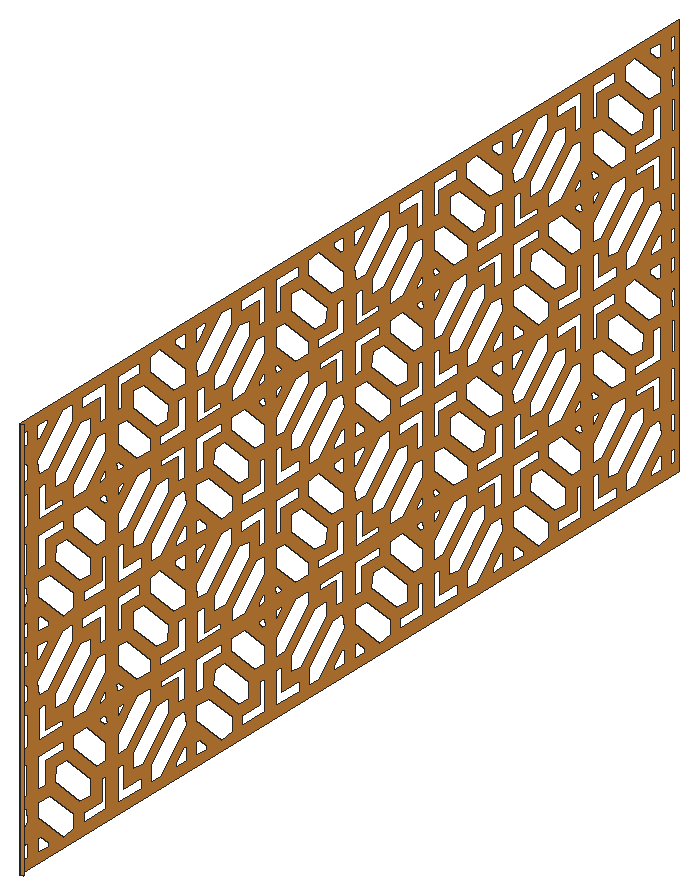
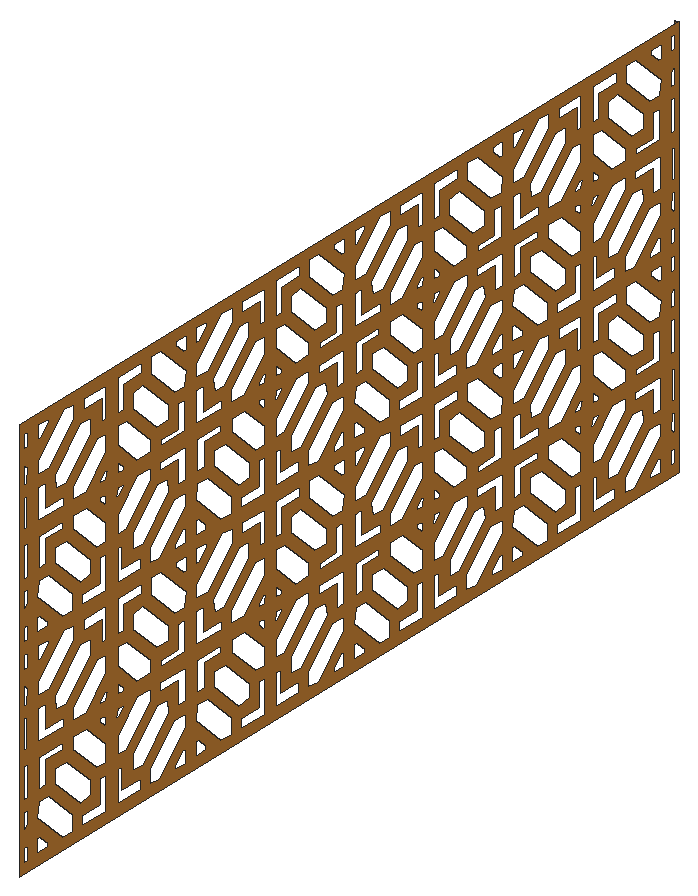
# SketchUp Ruby script. Lengths in inches.
U = 1.inch
M = Sketchup.active_model
def pt(a) = Geom::Point3d.new(a.map { |v| v * U })
def face(e, loops, mat)
  f = e.add_face(loops[0].map { |a| pt(a) })
  loops[1..].each { |l| e.add_face(l.map { |a| pt(a) }).erase! }
  f.material = f.back_material = mat if mat
  f
end
# faces: each face lists its corners as indices into pts; further lists are holes
def faces(e, pts, list, mat = nil) = list.each { |f| face(e, (f[0].is_a?(Array) ? f : [f]).map { |l| l.map { |i| pts[i] } }, mat) }
# xy, xz, yz: faces in a plane at the given z, y or x. An outline is a flat list of corners, or four numbers for a rectangle; further outlines are holes
def ring(l) = l.size == 4 ? [[l[0], l[1]], [l[2], l[1]], [l[2], l[3]], [l[0], l[3]]] : l.each_slice(2).to_a
def flat(e, list, mat, &to3) = list.each { |f| face(e, (f[0].is_a?(Array) ? f : [f]).map { |l| ring(l).map { |u, v| to3.(u, v) } }, mat) }
def xy(e, z, list, mat = nil) = flat(e, list, mat) { |x, y| [x, y, z] }
def xz(e, y, list, mat = nil) = flat(e, list, mat) { |x, z| [x, y, z] }
def yz(e, x, list, mat = nil) = flat(e, list, mat) { |y, z| [x, y, z] }
def lines(e, pts, list) = list.each { |a, b| e.add_line(pt(pts[a]), pt(pts[b])) }
# prism: a flat outline (further loops are holes) pulled along v
def prism(e, loops, v, mat = nil)
  f = face(e, loops, mat); d = Geom::Vector3d.new(v.map { |x| x * U })
  f.pushpull(f.normal.samedirection?(d) ? d.length : -d.length)
end
def box(e, o, s, mat = nil) = prism(e, [[o, [o[0] + s[0], o[1], o[2]], [o[0] + s[0], o[1] + s[1], o[2]], [o[0], o[1] + s[1], o[2]]]], [0, 0, s[2]], mat)
def at(x, y, z, deg = 0) = Geom::Transformation.translation(pt([x, y, z])) * Geom::Transformation.rotation(ORIGIN, Z_AXIS, deg.degrees)
def axes(o, x, y, z) = Geom::Transformation.new([*x, 0, *y, 0, *z, 0, *pt(o).to_a, 1])
def part(name) = M.definitions.add(name)
# library, detail: a bought-in or finely detailed component or shape, given as its bounding box
def library(name, o, s) = part(name).tap { |d| box(d.entities, o, s) }
def detail(e, o, s) = box(e.add_group.entities, o, s)
def put(e, d, t, mat = nil) = e.add_instance(d, t).tap { |i| i.material = mat if mat }
def group(e, t, mat = nil) = e.add_group.tap { |g| g.transformation = t; g.material = mat if mat }.entities
root = M.entities
M.materials.add("1056 AP 9903 Mellow Melon-N").color = [219, 142, 59]
xz(root,13.79,[[14.35,145.75,15.0625,238.4375]],"1056 AP 9903 Mellow Melon-N")
yz(root,14.35,[[[13.79,145.75,202.3125,238.4375],[94.27,153.04,101.6,160.37,101.6,163.43,98.2,163.43,91.29,156.53,91.29,153.47],[94.27,198.38,101.6,205.71,101.6,208.78,98.2,208.78,91.29,201.875,91.29,198.8125],[23.81,175.41,27.21,175.41,34.12,182.3125,34.12,185.375,31.14,185.81,23.81,178.47],[69.15,175.41,72.56,175.41,79.46,182.3125,79.46,185.375,76.48,185.81,69.15,178.47],[69.15,220.75,72.56,220.75,79.46,227.66,79.46,230.72,76.48,231.15,69.15,223.82],[23.81,220.75,27.21,220.75,34.12,227.66,34.12,230.72,31.14,231.15,23.81,223.82],[159.84,220.75,163.24,220.75,170.15,227.66,170.15,230.72,167.17,231.15,159.84,223.82],[159.84,175.41,163.24,175.41,170.15,182.3125,170.15,185.375,167.17,185.81,159.84,178.47],[48.93,153.04,56.26,160.37,56.26,163.43,52.85,163.43,45.95,156.53,45.95,153.47],[48.93,198.38,56.26,205.71,56.26,208.78,52.85,208.78,45.95,201.875,45.95,198.8125],[184.96,153.04,192.29,160.37,192.29,163.43,188.88,163.43,181.98,156.53,181.98,153.47],[139.62,153.04,146.95,160.37,146.95,163.43,143.54,163.43,136.64,156.53,136.64,153.47],[114.49,220.75,117.9,220.75,124.81,227.66,124.81,230.72,121.83,231.15,114.49,223.82],[114.49,175.41,117.9,175.41,124.81,182.3125,124.81,185.375,121.83,185.81,114.49,178.47],[139.62,198.38,146.95,205.71,146.95,208.78,143.54,208.78,136.64,201.875,136.64,198.8125],[184.96,198.38,192.29,205.71,192.29,208.78,188.88,208.78,181.98,201.875,181.98,198.8125],[98.27,175.34,101.33,175.34,101.76,178.32,94.43,185.65,91.36,185.65,91.36,182.24],[98.27,220.68,101.33,220.68,101.76,223.66,94.43,230.99,91.36,230.99,91.36,227.59],[52.92,175.34,55.99,175.34,56.42,178.32,49.09,185.65,46.02,185.65,46.02,182.24],[143.61,175.34,146.68,175.34,147.1,178.32,139.77,185.65,136.71,185.65,136.71,182.24],[30.98,198.54,34.05,198.54,34.05,201.95,27.14,208.85,24.08,208.85,23.65,205.87],[76.32,198.54,79.39,198.54,79.39,201.95,72.49,208.85,69.42,208.85,68.99,205.87],[52.92,220.68,55.99,220.68,56.42,223.66,49.09,230.99,46.02,230.99,46.02,227.59],[30.98,153.19,34.05,153.19,34.05,156.6,27.14,163.51,24.08,163.51,23.65,160.53],[76.32,153.19,79.39,153.19,79.39,156.6,72.49,163.51,69.42,163.51,68.99,160.53],[143.61,220.68,146.68,220.68,147.1,223.66,139.77,230.99,136.71,230.99,136.71,227.59],[188.96,175.34,192.02,175.34,192.45,178.32,185.12,185.65,182.05,185.65,182.05,182.24],[121.67,198.54,124.73,198.54,124.73,201.95,117.83,208.85,114.77,208.85,114.34,205.87],[167.01,198.54,170.08,198.54,170.08,201.95,163.17,208.85,160.11,208.85,159.68,205.87],[188.96,220.68,192.02,220.68,192.45,223.66,185.12,230.99,182.05,230.99,182.05,227.59],[121.67,153.19,124.73,153.19,124.73,156.6,117.83,163.51,114.77,163.51,114.34,160.53],[167.01,153.19,170.08,153.19,170.08,156.6,163.17,163.51,160.11,163.51,159.68,160.53],[96.45,148.27,99.42,148.27,106.76,155.61,106.33,158.67,103.35,158.67,96.45,151.76],[141.79,148.27,144.77,148.27,152.11,155.61,151.67,158.67,148.7,158.67,141.79,151.76],[96.45,193.61,99.42,193.61,106.76,200.95,106.33,204.01,103.35,204.01,96.45,197.11],[141.79,193.61,144.77,193.61,152.11,200.95,151.67,204.01,148.7,204.01,141.79,197.11],[187.14,148.27,190.11,148.27,197.45,155.61,197.02,158.67,194.04,158.67,187.14,151.76],[51.11,148.27,54.08,148.27,61.42,155.61,60.99,158.67,58.01,158.67,51.11,151.76],[187.14,193.61,190.11,193.61,197.45,200.95,197.02,204.01,194.04,204.01,187.14,197.11],[51.11,193.61,54.08,193.61,61.42,200.95,60.99,204.01,58.01,204.01,51.11,197.11],[193.72,180.49,197.22,180.49,197.22,183.47,189.88,190.81,186.82,190.375,186.82,187.4],[193.72,225.84,197.22,225.84,197.22,228.8125,189.88,236.15,186.82,235.72,186.82,232.74],[26.22,193.38,29.28,193.8125,29.28,196.79,22.375,203.69,18.88,203.69,18.88,200.72],[116.91,193.38,119.97,193.8125,119.97,196.79,113.0625,203.69,109.57,203.69,109.57,200.72],[162.25,193.38,165.3125,193.8125,165.3125,196.79,158.41,203.69,154.91,203.69,154.91,200.72],[71.5625,193.38,74.625,193.8125,74.625,196.79,67.72,203.69,64.22,203.69,64.22,200.72],[71.5625,148.03,74.625,148.47,74.625,151.45,67.72,158.35,64.22,158.35,64.22,155.375],[26.22,148.03,29.28,148.47,29.28,151.45,22.375,158.35,18.88,158.35,18.88,155.375],[116.91,148.03,119.97,148.47,119.97,151.45,113.0625,158.35,109.57,158.35,109.57,155.375],[162.25,148.03,165.3125,148.47,165.3125,151.45,158.41,158.35,154.91,158.35,154.91,155.375],[103.04,225.84,106.53,225.84,106.53,228.8125,99.19,236.15,96.13,235.72,96.13,232.74],[103.04,180.49,106.53,180.49,106.53,183.47,99.19,190.81,96.13,190.375,96.13,187.4],[148.38,225.84,151.875,225.84,151.875,228.8125,144.54,236.15,141.48,235.72,141.48,232.74],[148.38,180.49,151.875,180.49,151.875,183.47,144.54,190.81,141.48,190.375,141.48,187.4],[57.69,225.84,61.1875,225.84,61.1875,228.8125,53.85,236.15,50.79,235.72,50.79,232.74],[57.69,180.49,61.1875,180.49,61.1875,183.47,53.85,190.81,50.79,190.375,50.79,187.4],[109.77,180.18,112.75,180.18,119.65,187.08,119.65,190.58,116.67,190.58,109.33,183.24],[109.77,225.52,112.75,225.52,119.65,232.42,119.65,235.92,116.67,235.92,109.33,228.58],[155.11,225.52,158.09,225.52,164.99,232.42,164.99,235.92,162.02,235.92,154.68,228.58],[155.11,180.18,158.09,180.18,164.99,187.08,164.99,190.58,162.02,190.58,154.68,183.24],[64.42,225.52,67.4,225.52,74.31,232.42,74.31,235.92,71.33,235.92,63.99,228.58],[64.42,180.18,67.4,180.18,74.31,187.08,74.31,190.58,71.33,190.58,63.99,183.24],[19.08,180.18,22.06,180.18,28.96,187.08,28.96,190.58,25.99,190.58,18.65,183.24],[19.08,225.52,22.06,225.52,28.96,232.42,28.96,235.92,25.99,235.92,18.65,228.58],[28.96,216.42,32.8,216.42,38.41,222.03,38.41,225.95,35.87,225.95,28.96,219.05],[74.31,216.42,78.15,216.42,83.76,222.03,83.76,225.95,81.21,225.95,74.31,219.05],[74.31,171.08,78.15,171.08,83.76,176.68,83.76,180.61,81.21,180.61,74.31,173.71],[28.96,171.08,32.8,171.08,38.41,176.68,38.41,180.61,35.87,180.61,28.96,173.71],[119.65,216.42,123.49,216.42,129.1,222.03,129.1,225.95,126.55,225.95,119.65,219.05],[164.99,216.42,168.84,216.42,174.45,222.03,174.45,225.95,171.9,225.95,164.99,219.05],[164.99,171.08,168.84,171.08,174.45,176.68,174.45,180.61,171.9,180.61,164.99,173.71],[119.65,171.08,123.49,171.08,129.1,176.68,129.1,180.61,126.55,180.61,119.65,173.71],[47.3,216.39,51.22,216.39,51.22,218.93,44.32,225.84,41.6875,225.84,41.6875,221.99],[92.64,216.39,96.56,216.39,96.56,218.93,89.66,225.84,87.03,225.84,87.03,221.99],[183.33,216.39,187.25,216.39,187.25,218.93,180.35,225.84,177.72,225.84,177.72,221.99],[137.98,216.39,141.91,216.39,141.91,218.93,135,225.84,132.375,225.84,132.375,221.99],[47.3,171.04,51.22,171.04,51.22,173.59,44.32,180.49,41.6875,180.49,41.6875,176.65],[183.33,171.04,187.25,171.04,187.25,173.59,180.35,180.49,177.72,180.49,177.72,176.65],[92.64,171.04,96.56,171.04,96.56,173.59,89.66,180.49,87.03,180.49,87.03,176.65],[137.98,171.04,141.91,171.04,141.91,173.59,135,180.49,132.375,180.49,132.375,176.65],[35.75,203.69,38.38,203.69,38.38,207.54,32.77,213.15,28.85,213.15,28.85,210.6],[35.75,158.35,38.38,158.35,38.38,162.19,32.77,167.8,28.85,167.8,28.85,165.25],[81.09,203.69,83.72,203.69,83.72,207.54,78.11,213.15,74.19,213.15,74.19,210.6],[171.78,203.69,174.41,203.69,174.41,207.54,168.8,213.15,164.88,213.15,164.88,210.6],[81.09,158.35,83.72,158.35,83.72,162.19,78.11,167.8,74.19,167.8,74.19,165.25],[126.4375,203.69,129.07,203.69,129.07,207.54,123.46,213.15,119.53,213.15,119.53,210.6],[171.78,158.35,174.41,158.35,174.41,162.19,168.8,167.8,164.88,167.8,164.88,165.25],[126.4375,158.35,129.07,158.35,129.07,162.19,123.46,167.8,119.53,167.8,119.53,165.25],[132.34,203.58,134.89,203.58,141.79,210.48,141.79,213.11,137.95,213.11,132.34,207.5],[87,203.58,89.54,203.58,96.45,210.48,96.45,213.11,92.61,213.11,87,207.5],[132.34,158.23,134.89,158.23,141.79,165.14,141.79,167.77,137.95,167.77,132.34,162.16],[41.65,203.58,44.2,203.58,51.11,210.48,51.11,213.11,47.26,213.11,41.65,207.5],[87,158.23,89.54,158.23,96.45,165.14,96.45,167.77,92.61,167.77,87,162.16],[41.65,158.23,44.2,158.23,51.11,165.14,51.11,167.77,47.26,167.77,41.65,162.16],[177.68,203.58,180.23,203.58,187.14,210.48,187.14,213.11,183.29,213.11,177.68,207.5],[177.68,158.23,180.23,158.23,187.14,165.14,187.14,167.77,183.29,167.77,177.68,162.16],[132.34,148.27,139.21,148.27,139.21,150.43,134.06,150.43,134.06,155.63,132.34,155.63],[132.34,193.61,139.21,193.61,139.21,195.78,134.06,195.78,134.06,200.98,132.34,200.98],[36.7,183.21,38.41,183.21,38.41,190.58,31.54,190.58,31.54,188.41,36.7,188.41],[87,148.27,93.87,148.27,93.87,150.43,88.72,150.43,88.72,155.63,87,155.63],[172.73,183.21,174.45,183.21,174.45,190.58,167.57,190.58,167.57,188.41,172.73,188.41],[177.68,148.27,184.56,148.27,184.56,150.43,179.4,150.43,179.4,155.63,177.68,155.63],[36.7,228.55,38.41,228.55,38.41,235.92,31.54,235.92,31.54,233.75,36.7,233.75],[87,193.61,93.87,193.61,93.87,195.78,88.72,195.78,88.72,200.98,87,200.98],[82.04,183.21,83.76,183.21,83.76,190.58,76.88,190.58,76.88,188.41,82.04,188.41],[41.65,148.27,48.53,148.27,48.53,150.43,43.37,150.43,43.37,155.63,41.65,155.63],[177.68,193.61,184.56,193.61,184.56,195.78,179.4,195.78,179.4,200.98,177.68,200.98],[172.73,228.55,174.45,228.55,174.45,235.92,167.57,235.92,167.57,233.75,172.73,233.75],[41.65,193.61,48.53,193.61,48.53,195.78,43.37,195.78,43.37,200.98,41.65,200.98],[82.04,228.55,83.76,228.55,83.76,235.92,76.88,235.92,76.88,233.75,82.04,233.75],[127.38,183.21,129.1,183.21,129.1,190.58,122.23,190.58,122.23,188.41,127.38,188.41],[127.38,228.55,129.1,228.55,129.1,235.92,122.23,235.92,122.23,233.75,127.38,233.75],[189.85,216.39,197.22,216.39,197.22,223.26,195.05,223.26,195.05,218.1,189.85,218.1],[109.57,206.27,111.73,206.27,111.73,211.43,116.93,211.43,116.93,213.15,109.57,213.15],[99.16,216.39,106.53,216.39,106.53,223.26,104.37,223.26,104.37,218.1,99.16,218.1],[144.51,216.39,151.875,216.39,151.875,223.26,149.71,223.26,149.71,218.1,144.51,218.1],[53.82,216.39,61.1875,216.39,61.1875,223.26,59.02,223.26,59.02,218.1,53.82,218.1],[154.91,206.27,157.08,206.27,157.08,211.43,162.28,211.43,162.28,213.15,154.91,213.15],[189.85,171.04,197.22,171.04,197.22,177.92,195.05,177.92,195.05,172.76,189.85,172.76],[99.16,171.04,106.53,171.04,106.53,177.92,104.37,177.92,104.37,172.76,99.16,172.76],[144.51,171.04,151.875,171.04,151.875,177.92,149.71,177.92,149.71,172.76,144.51,172.76],[109.57,160.93,111.73,160.93,111.73,166.08,116.93,166.08,116.93,167.8,109.57,167.8],[53.82,171.04,61.1875,171.04,61.1875,177.92,59.02,177.92,59.02,172.76,53.82,172.76],[154.91,160.93,157.08,160.93,157.08,166.08,162.28,166.08,162.28,167.8,154.91,167.8],[64.22,206.27,66.39,206.27,66.39,211.43,71.59,211.43,71.59,213.15,64.22,213.15],[18.88,206.27,21.05,206.27,21.05,211.43,26.25,211.43,26.25,213.15,18.88,213.15],[64.22,160.93,66.39,160.93,66.39,166.08,71.59,166.08,71.59,167.8,64.22,167.8],[18.88,160.93,21.05,160.93,21.05,166.08,26.25,166.08,26.25,167.8,18.88,167.8],[31.88,193.8125,38.38,193.8125,38.38,200.6875,37.08,200.6875,37.08,195.96,31.88,195.96],[31.88,148.47,38.38,148.47,38.38,155.34,37.08,155.34,37.08,150.62,31.88,150.62],[87.03,228.84,88.33,228.84,88.33,233.57,93.53,233.57,93.53,235.72,87.03,235.72],[41.6875,228.84,42.99,228.84,42.99,233.57,48.1875,233.57,48.1875,235.72,41.6875,235.72],[41.6875,183.5,42.99,183.5,42.99,188.23,48.1875,188.23,48.1875,190.375,41.6875,190.375],[87.03,183.5,88.33,183.5,88.33,188.23,93.53,188.23,93.53,190.375,87.03,190.375],[77.22,148.47,83.72,148.47,83.72,155.34,82.42,155.34,82.42,150.62,77.22,150.62],[77.22,193.8125,83.72,193.8125,83.72,200.6875,82.42,200.6875,82.42,195.96,77.22,195.96],[177.72,183.5,179.02,183.5,179.02,188.23,184.22,188.23,184.22,190.375,177.72,190.375],[132.375,183.5,133.67,183.5,133.67,188.23,138.875,188.23,138.875,190.375,132.375,190.375],[122.57,148.47,129.07,148.47,129.07,155.34,127.77,155.34,127.77,150.62,122.57,150.62],[122.57,193.8125,129.07,193.8125,129.07,200.6875,127.77,200.6875,127.77,195.96,122.57,195.96],[167.91,193.8125,174.41,193.8125,174.41,200.6875,173.11,200.6875,173.11,195.96,167.91,195.96],[167.91,148.47,174.41,148.47,174.41,155.34,173.11,155.34,173.11,150.62,167.91,150.62],[177.72,228.84,179.02,228.84,179.02,233.57,184.22,233.57,184.22,235.72,177.72,235.72],[132.375,228.84,133.67,228.84,133.67,233.57,138.875,233.57,138.875,235.72,132.375,235.72],[194.87,206.61,197.02,206.61,197.02,213.11,190.14,213.11,190.14,211.8125,194.87,211.8125],[19.08,216.42,25.95,216.42,25.95,217.72,21.23,217.72,21.23,222.92,19.08,222.92],[194.87,161.27,197.02,161.27,197.02,167.77,190.14,167.77,190.14,166.47,194.87,166.47],[104.18,206.61,106.33,206.61,106.33,213.11,99.46,213.11,99.46,211.8125,104.18,211.8125],[19.08,171.08,25.95,171.08,25.95,172.375,21.23,172.375,21.23,177.58,19.08,177.58],[109.77,216.42,116.64,216.42,116.64,217.72,111.92,217.72,111.92,222.92,109.77,222.92],[155.11,216.42,161.99,216.42,161.99,217.72,157.26,217.72,157.26,222.92,155.11,222.92],[104.18,161.27,106.33,161.27,106.33,167.77,99.46,167.77,99.46,166.47,104.18,166.47],[64.42,216.42,71.3,216.42,71.3,217.72,66.57,217.72,66.57,222.92,64.42,222.92],[58.84,206.61,60.99,206.61,60.99,213.11,54.11,213.11,54.11,211.8125,58.84,211.8125],[149.53,206.61,151.67,206.61,151.67,213.11,144.8,213.11,144.8,211.8125,149.53,211.8125],[109.77,171.08,116.64,171.08,116.64,172.375,111.92,172.375,111.92,177.58,109.77,177.58],[155.11,171.08,161.99,171.08,161.99,172.375,157.26,172.375,157.26,177.58,155.11,177.58],[58.84,161.27,60.99,161.27,60.99,167.77,54.11,167.77,54.11,166.47,58.84,166.47],[64.42,171.08,71.3,171.08,71.3,172.375,66.57,172.375,66.57,177.58,64.42,177.58],[149.53,161.27,151.67,161.27,151.67,167.77,144.8,167.77,144.8,166.47,149.53,166.47],[200.25,206.27,201.3125,213.15],[200.25,160.93,201.3125,167.8],[14.79,216.39,15.84,223.26],[14.79,171.04,15.84,177.92],[58.41,148.27,61.42,148.27,61.42,151.3,60.57,151.3,58.41,149.14],[58.41,193.61,61.42,193.61,61.42,196.64,60.57,196.64,58.41,194.49],[149.1,148.27,152.1,148.27,152.1,151.3,151.25,151.3,149.1,149.14],[103.75,148.27,106.76,148.27,106.76,151.3,105.91,151.3,103.75,149.14],[194.44,148.27,197.45,148.27,197.45,151.3,196.6,151.3,194.44,149.14],[103.75,193.61,106.76,193.61,106.76,196.64,105.91,196.64,103.75,194.49],[149.1,193.61,152.1,193.61,152.1,196.64,151.25,196.64,149.1,194.49],[194.44,193.61,197.45,193.61,197.45,196.64,196.6,196.64,194.44,194.49],[18.88,193.38,21.91,193.38,21.91,194.23,19.75,196.39,18.88,196.39],[64.22,193.38,67.26,193.38,67.26,194.23,65.1,196.39,64.22,196.39],[109.57,193.38,112.6,193.38,112.6,194.23,110.44,196.39,109.57,196.39],[154.91,193.38,157.94,193.38,157.94,194.23,155.79,196.39,154.91,196.39],[64.22,148.04,67.26,148.04,67.26,148.89,65.1,151.05,64.22,151.05],[18.88,148.04,21.91,148.04,21.91,148.89,19.75,151.05,18.88,151.05],[154.91,148.04,157.94,148.04,157.94,148.89,155.79,151.05,154.91,151.05],[109.57,148.04,112.6,148.04,112.6,148.89,110.44,151.05,109.57,151.05],[196.34,233.14,197.22,233.14,197.22,236.15,194.1875,236.15,194.1875,235.3],[196.34,187.8,197.22,187.8,197.22,190.8,194.1875,190.8,194.1875,189.95],[151,233.14,151.875,233.14,151.875,236.15,148.84,236.15,148.84,235.3],[151,187.8,151.875,187.8,151.875,190.8,148.84,190.8,148.84,189.95],[105.66,233.14,106.53,233.14,106.53,236.15,103.5,236.15,103.5,235.3],[105.66,187.8,106.53,187.8,106.53,190.8,103.5,190.8,103.5,189.95],[60.3125,233.14,61.1875,233.14,61.1875,236.15,58.15,236.15,58.15,235.3],[60.3125,187.8,61.1875,187.8,61.1875,190.8,58.15,190.8,58.15,189.95],[63.99,187.54,64.84,187.54,67,189.7,67,190.58,63.99,190.58],[63.99,232.89,64.84,232.89,67,235.04,67,235.92,63.99,235.92],[109.34,187.54,110.1875,187.54,112.35,189.7,112.35,190.58,109.34,190.58],[109.34,232.89,110.1875,232.89,112.35,235.04,112.35,235.92,109.34,235.92],[154.68,232.89,155.53,232.89,157.6875,235.04,157.6875,235.92,154.68,235.92],[154.68,187.54,155.53,187.54,157.6875,189.7,157.6875,190.58,154.68,190.58],[18.65,187.54,19.5,187.54,21.66,189.7,21.66,190.58,18.65,190.58],[18.65,232.89,19.5,232.89,21.66,235.04,21.66,235.92,18.65,235.92],[200.46,216.42,201.3125,222.92],[200.46,171.08,201.3125,177.58],[14.79,206.61,15.64,213.11],[14.79,161.27,15.64,167.77],[200.46,225.52,201.3125,225.52,201.3125,229.87,200.02,228.58],[200.46,180.18,201.3125,180.18,201.3125,184.53,200.02,183.24],[14.79,154.31,16.08,155.61,15.64,158.67,14.79,158.67],[14.79,199.66,16.08,200.95,15.64,204.01,14.79,204.01],[14.79,148.27,16.07,148.27,16.07,151.3,15.22,151.3,14.79,150.86],[14.79,193.61,16.07,193.61,16.07,196.64,15.22,196.64,14.79,196.21],[200.03,232.89,200.875,232.89,201.3125,233.32,201.3125,235.92,200.03,235.92],[200.03,187.54,200.875,187.54,201.3125,187.98,201.3125,190.58,200.03,190.58],[201.3125,199.66,201.3125,203.69,200.25,203.69,200.25,200.72],[201.3125,154.31,201.3125,158.35,200.25,158.35,200.25,155.375],[14.79,225.84,15.84,225.84,15.84,228.8125,14.79,229.87],[14.79,180.49,15.84,180.49,15.84,183.47,14.79,184.53],[14.97,233.14,15.84,233.14,15.84,236.15,14.79,236.15,14.79,233.32],[14.97,187.8,15.84,187.8,15.84,190.8,14.79,190.8,14.79,187.98],[200.25,193.38,201.3125,193.38,201.3125,196.21,201.13,196.39,200.25,196.39],[200.25,148.04,201.3125,148.04,201.3125,150.86,201.13,151.05,200.25,151.05],[36.7,215.99,38.41,216.42,38.41,218.15,37.99,218.15,36.7,216.86],[172.73,215.99,174.45,216.42,174.45,218.15,174.02,218.15,172.73,216.86],[36.7,170.64,38.41,171.08,38.41,172.81,37.99,172.81,36.7,171.51],[172.73,170.64,174.45,171.08,174.45,172.81,174.02,172.81,172.73,171.51],[82.04,215.99,83.76,216.42,83.76,218.15,83.33,218.15,82.04,216.86],[82.04,170.64,83.76,171.08,83.76,172.81,83.33,172.81,82.04,171.51],[127.38,215.99,129.1,216.42,129.1,218.15,128.68,218.15,127.38,216.86],[127.38,170.64,129.1,171.08,129.1,172.81,128.68,172.81,127.38,171.51],[177.72,216.39,179.45,216.39,179.45,216.81,178.16,218.1,177.28,218.1],[41.6875,216.39,43.42,216.39,43.42,216.81,42.125,218.1,41.25,218.1],[37.94,211.43,38.8125,211.43,38.38,213.15,36.65,213.15,36.65,212.72],[132.375,216.39,134.11,216.39,134.11,216.81,132.8125,218.1,131.94,218.1],[83.29,211.43,84.16,211.43,83.72,213.15,81.99,213.15,81.99,212.72],[173.97,211.43,174.84,211.43,174.41,213.15,172.68,213.15,172.68,212.72],[87.03,216.39,88.76,216.39,88.76,216.81,87.47,218.1,86.6,218.1],[177.72,171.04,179.45,171.04,179.45,171.47,178.16,172.76,177.28,172.76],[41.6875,171.04,43.42,171.04,43.42,171.47,42.125,172.76,41.25,172.76],[128.63,211.43,129.5,211.43,129.07,213.15,127.33,213.15,127.33,212.72],[37.94,166.08,38.8125,166.08,38.38,167.8,36.65,167.8,36.65,167.38],[132.375,171.04,134.11,171.04,134.11,171.47,132.8125,172.76,131.94,172.76],[83.29,166.08,84.16,166.08,83.72,167.8,81.99,167.8,81.99,167.38],[173.97,166.08,174.84,166.08,174.41,167.8,172.68,167.8,172.68,167.38],[87.03,171.04,88.76,171.04,88.76,171.47,87.47,172.76,86.6,172.76],[128.63,166.08,129.5,166.08,129.07,167.8,127.33,167.8,127.33,167.38],[132.34,211.38,132.76,211.38,134.06,212.67,134.06,213.55,132.34,213.11],[177.68,211.38,178.11,211.38,179.4,212.67,179.4,213.55,177.68,213.11],[132.34,166.04,132.76,166.04,134.06,167.33,134.06,168.2,132.34,167.77],[177.68,166.04,178.11,166.04,179.4,167.33,179.4,168.2,177.68,167.77],[87,211.38,87.42,211.38,88.72,212.67,88.72,213.55,87,213.11],[41.65,211.38,42.08,211.38,43.37,212.67,43.37,213.55,41.65,213.11],[87,166.04,87.42,166.04,88.72,167.33,88.72,168.2,87,167.77],[41.65,166.04,42.08,166.04,43.37,167.33,43.37,168.2,41.65,167.77]]],"1056 AP 9903 Mellow Melon-N")
